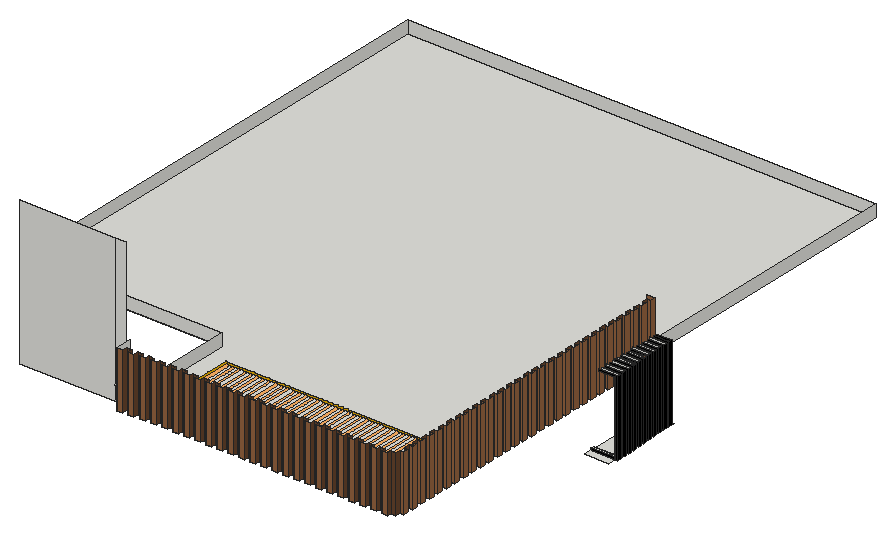
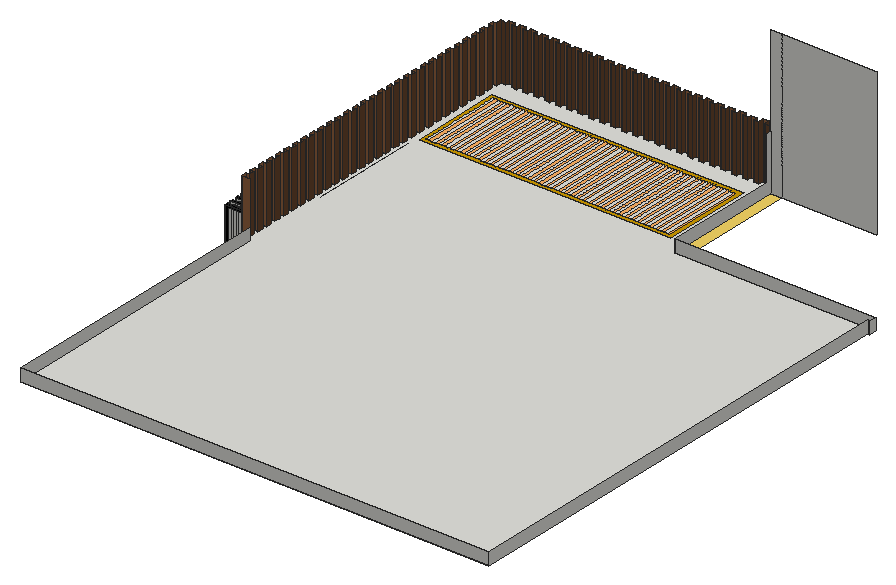
# SketchUp Ruby script. Lengths in inches.
U = 1.inch
M = Sketchup.active_model
def pt(a) = Geom::Point3d.new(a.map { |v| v * U })
def face(e, loops, mat)
  f = e.add_face(loops[0].map { |a| pt(a) })
  loops[1..].each { |l| e.add_face(l.map { |a| pt(a) }).erase! }
  f.material = f.back_material = mat if mat
  f
end
# faces: each face lists its corners as indices into pts; further lists are holes
def faces(e, pts, list, mat = nil) = list.each { |f| face(e, (f[0].is_a?(Array) ? f : [f]).map { |l| l.map { |i| pts[i] } }, mat) }
# xy, xz, yz: faces in a plane at the given z, y or x. An outline is a flat list of corners, or four numbers for a rectangle; further outlines are holes
def ring(l) = l.size == 4 ? [[l[0], l[1]], [l[2], l[1]], [l[2], l[3]], [l[0], l[3]]] : l.each_slice(2).to_a
def flat(e, list, mat, &to3) = list.each { |f| face(e, (f[0].is_a?(Array) ? f : [f]).map { |l| ring(l).map { |u, v| to3.(u, v) } }, mat) }
def xy(e, z, list, mat = nil) = flat(e, list, mat) { |x, y| [x, y, z] }
def xz(e, y, list, mat = nil) = flat(e, list, mat) { |x, z| [x, y, z] }
def yz(e, x, list, mat = nil) = flat(e, list, mat) { |y, z| [x, y, z] }
def lines(e, pts, list) = list.each { |a, b| e.add_line(pt(pts[a]), pt(pts[b])) }
# prism: a flat outline (further loops are holes) pulled along v
def prism(e, loops, v, mat = nil)
  f = face(e, loops, mat); d = Geom::Vector3d.new(v.map { |x| x * U })
  f.pushpull(f.normal.samedirection?(d) ? d.length : -d.length)
end
def box(e, o, s, mat = nil) = prism(e, [[o, [o[0] + s[0], o[1], o[2]], [o[0] + s[0], o[1] + s[1], o[2]], [o[0], o[1] + s[1], o[2]]]], [0, 0, s[2]], mat)
def at(x, y, z, deg = 0) = Geom::Transformation.translation(pt([x, y, z])) * Geom::Transformation.rotation(ORIGIN, Z_AXIS, deg.degrees)
def axes(o, x, y, z) = Geom::Transformation.new([*x, 0, *y, 0, *z, 0, *pt(o).to_a, 1])
def part(name) = M.definitions.add(name)
# library, detail: a bought-in or finely detailed component or shape, given as its bounding box
def library(name, o, s) = part(name).tap { |d| box(d.entities, o, s) }
def detail(e, o, s) = box(e.add_group.entities, o, s)
def put(e, d, t, mat = nil) = e.add_instance(d, t).tap { |i| i.material = mat if mat }
def group(e, t, mat = nil) = e.add_group.tap { |g| g.transformation = t; g.material = mat if mat }.entities
root = M.entities
M.materials.add("C03_Honey_Glow").color = [255, 178, 101]
M.materials.add("D06_Sunflower_Bright").color = [204, 153, 0]
M.materials.add("Glass_Mirror_3").color = [244, 212, 100]
M.materials.add("M09_Shadow_Night").color = [0, 0, 0]
M.materials.add("Wood_Veneer_15_1K").color = [150, 100, 65]
M.materials.add("Wood_Veneer_15_1K1").color = [103, 69, 45]
xy(root,467.31,[[444,372.3125,463.47,378.77],[463.47,378.77,466.08,381.22],[444,381.22,463.47,381.22,463.47,384.31,463.21,384.31,463.21,386.76,463.47,386.76,463.47,389.85,462.95,389.85,462.95,392.29,463.47,392.29,463.47,395.39,462.69,395.39,462.69,397.83,463.47,397.83,463.47,400.92,462.43,400.92,462.43,403.37,463.47,403.37,463.47,406.46,462.17,406.46,462.17,408.91,463.47,408.91,463.47,412,461.91,412,461.91,414.45,463.47,414.45,463.47,417.54,461.65,417.54,461.65,419.99,463.47,419.99,463.47,423.08,461.39,423.08,461.39,425.52,463.47,425.52,463.47,428.62,461.125,428.62,461.125,431.0625,463.47,431.0625,463.47,434.15,460.87,434.15,460.87,436.6,463.47,436.6,463.47,438.64,444,438.64],[463.21,384.31,463.47,386.76],[463.47,384.31,465.82,386.76],
  [462.95,389.85,463.47,392.29],[463.47,389.85,465.56,392.29],[462.69,395.39,463.47,397.83],[463.47,395.39,465.3,397.83],[462.43,400.92,463.47,403.37],
  [463.47,400.92,465.04,403.37],[462.17,406.46,463.47,408.91],[463.47,406.46,464.78,408.91],[461.91,412,463.47,414.45],[463.47,412,464.51,414.45],
  [461.65,417.54,463.47,419.99],[463.47,417.54,464.25,419.99],[461.39,423.08,463.47,425.52],[463.47,423.08,463.99,425.52],[461.125,428.62,463.47,431.0625],
  [463.47,428.62,463.73,431.0625],[460.87,434.15,463.47,436.6]])
xy(root,468.96,[[444,378.77,463.47,381.22]])
xy(root,509.54,[[[222,171,222,278.44,57.3,278.44,57.3,284.23,59.5,284.23,59.5,671.23,443.5,671.23,443.5,436.68,449.91,436.68,449.91,432.33,446.91,432.33,446.91,427.97,449.91,427.97,449.91,423.61,446.91,423.61,446.91,419.25,449.91,419.25,449.91,414.89,446.91,414.89,446.91,410.54,449.91,410.54,449.91,406.18,446.91,406.18,446.91,401.82,449.91,401.82,449.91,397.46,446.91,397.46,446.91,393.11,449.91,393.11,449.91,388.75,446.91,388.75,446.91,384.39,449.91,384.39,449.91,380.03,446.91,380.03,446.91,375.68,449.91,375.68,449.91,371.32,446.91,371.32,446.91,366.96,449.91,366.96,449.91,362.6,446.91,362.6,446.91,358.25,449.91,358.25,449.91,353.89,446.91,353.89,446.91,349.53,449.91,349.53,449.91,345.17,446.91,345.17,446.91,340.82,449.91,340.82,449.91,336.46,446.91,336.46,446.91,332.1,449.91,332.1,449.91,327.74,446.91,327.74,446.91,323.38,449.91,323.38,449.91,319.03,446.91,319.03,446.91,314.67,449.91,314.67,449.91,310.3125,446.91,310.3125,446.91,305.95,449.91,305.95,449.91,301.6,446.91,301.6,446.91,297.24,449.91,297.24,449.91,292.88,446.91,292.88,446.91,288.52,449.91,288.52,449.91,284.17,446.91,284.17,446.91,279.81,449.91,279.81,449.91,275.45,446.91,275.45,446.91,271.09,449.91,271.09,449.91,266.74,446.91,266.74,446.91,262.38,449.91,262.38,449.91,258.02,446.91,258.02,446.91,253.66,449.91,253.66,449.91,249.31,446.91,249.31,446.91,244.95,449.91,244.95,449.91,240.59,446.91,240.59,446.91,236.23,449.91,236.23,449.91,231.875,446.91,231.875,446.91,227.52,449.91,227.52,449.91,223.16,446.91,223.16,446.91,218.8,449.91,218.8,449.91,214.44,446.91,214.44,446.91,210.09,449.91,210.09,449.91,205.73,446.91,205.73,446.91,201.37,449.91,201.37,449.91,197.01,446.91,197.01,446.91,192.66,449.91,192.66,449.91,188.3,446.91,188.3,446.91,183.94,449.91,183.94,449.91,179.58,446.91,179.58,446.91,175.23,442.41,175.23,442.41,172.23,437.91,172.23,437.91,175.23,433.42,175.23,433.42,172.23,428.92,172.23,428.92,175.23,424.42,175.23,424.42,172.23,419.92,172.23,419.92,175.23,415.42,175.23,415.42,172.23,410.92,172.23,410.92,175.23,406.43,175.23,406.43,172.23,401.93,172.23,401.93,175.23,397.43,175.23,397.43,172.23,392.93,172.23,392.93,175.23,388.43,175.23,388.43,172.23,383.9375,172.23,383.9375,175.23,379.4375,175.23,379.4375,172.23,374.9375,172.23,374.9375,175.23,370.44,175.23,370.44,172.23,365.94,172.23,365.94,175.23,361.44,175.23,361.44,172.23,356.95,172.23,356.95,175.23,352.45,175.23,352.45,172.23,347.95,172.23,347.95,175.23,343.45,175.23,343.45,172.23,338.95,172.23,338.95,175.23,334.46,175.23,334.46,172.23,329.96,172.23,329.96,175.23,325.46,175.23,325.46,172.23,320.96,172.23,320.96,175.23,316.46,175.23,316.46,172.23,311.96,172.23,311.96,175.23,307.47,175.23,307.47,172.23,302.97,172.23,302.97,175.23,298.47,175.23,298.47,172.23,293.97,172.23,293.97,175.23,289.47,175.23,289.47,172.23,284.97,172.23,284.97,175.23,280.48,175.23,280.48,172.23,275.98,172.23,275.98,175.23,271.48,175.23,271.48,172.23,266.98,172.23,266.98,175.23,262.48,175.23,262.48,172.23,257.99,172.23,257.99,175.23,253.49,175.23,253.49,172.23,248.99,172.23,248.99,175.23,244.49,175.23,244.49,172.23,239.99,172.23,239.99,175.23,235.49,175.23,235.49,171,231,171,231,175.23,226.5,175.23,226.5,171],[235.75,190.61,441.53,265.07]],[241.25,193.61,243.74,262.07],[246.24,193.61,248.74,262.07],[251.24,193.61,253.73,262.07],[256.23,193.61,258.73,262.07],
  [261.22,193.61,263.72,262.07],[266.22,193.61,268.72,262.07],[271.21,193.61,273.71,262.07],[276.21,193.61,278.71,262.07],[281.2,193.61,283.7,262.07],
  [286.2,193.61,288.69,262.07],[291.19,193.61,293.6875,262.07],[296.1875,193.61,298.68,262.07],[301.18,193.61,303.68,262.07],[306.17,193.61,308.67,262.07],
  [311.17,193.61,313.67,262.07],[316.16,193.61,318.66,262.07],[321.16,193.61,323.65,262.07],[326.15,193.61,328.65,262.07],[331.15,193.61,333.64,262.07],
  [336.14,193.61,338.64,262.07],[341.14,193.61,343.63,262.07],[346.13,193.61,348.625,262.07],[351.125,193.61,353.62,262.07],[356.12,193.61,358.62,262.07],
  [361.11,193.61,363.61,262.07],[366.11,193.61,368.6,262.07],[371.1,193.61,373.6,262.07],[376.1,193.61,378.59,262.07],[381.09,193.61,383.59,262.07],
  [386.09,193.61,388.58,262.07],[391.08,193.61,393.58,262.07],[396.07,193.61,398.57,262.07],[401.07,193.61,403.57,262.07],[406.0625,193.61,408.56,262.07],
  [411.06,193.61,413.55,262.07],[416.05,193.61,418.55,262.07],[421.05,193.61,423.54,262.07],[426.04,193.61,428.54,262.07],[431.03,193.61,433.53,262.07],
  [436.03,193.61,438.53,262.07]])
xy(root,509.54,[[238.75,193.61,241.25,262.07],[243.74,193.61,246.24,262.07],[248.74,193.61,251.24,262.07],[253.73,193.61,256.23,262.07],[258.73,193.61,261.22,262.07],
  [263.72,193.61,266.22,262.07],[268.72,193.61,271.21,262.07],[273.71,193.61,276.21,262.07],[278.71,193.61,281.2,262.07],[283.7,193.61,286.2,262.07],
  [288.69,193.61,291.19,262.07],[293.6875,193.61,296.1875,262.07],[298.68,193.61,301.18,262.07],[303.68,193.61,306.17,262.07],[308.67,193.61,311.17,262.07],
  [313.67,193.61,316.16,262.07],[318.66,193.61,321.16,262.07],[323.65,193.61,326.15,262.07],[328.65,193.61,331.15,262.07],[333.64,193.61,336.14,262.07],
  [338.64,193.61,341.14,262.07],[343.63,193.61,346.13,262.07],[348.625,193.61,351.125,262.07],[353.62,193.61,356.12,262.07],[358.62,193.61,361.11,262.07],
  [363.61,193.61,366.11,262.07],[368.6,193.61,371.1,262.07],[373.6,193.61,376.1,262.07],[378.59,193.61,381.09,262.07],[383.59,193.61,386.09,262.07],
  [388.58,193.61,391.08,262.07],[393.58,193.61,396.07,262.07],[398.57,193.61,401.07,262.07],[403.57,193.61,406.0625,262.07],[408.56,193.61,411.06,262.07],
  [413.55,193.61,416.05,262.07],[418.55,193.61,421.05,262.07],[423.54,193.61,426.04,262.07],[428.54,193.61,431.03,262.07],[433.53,193.61,436.03,262.07]],"C03_Honey_Glow")
xy(root,509.54,[[[235.75,190.61,441.53,265.07],[238.75,193.61,438.53,262.07]]],"D06_Sunflower_Bright")
xy(root,509.54,[[213,180,222,272.89]],"Glass_Mirror_3")
xz(root,171,[[222,509.54,226.5,555.54],[231,509.54,235.49,555.54]],"Wood_Veneer_15_1K")
xz(root,172.23,[[239.99,509.54,244.49,555.54],[248.99,509.54,253.49,555.54],[257.99,509.54,262.48,555.54],[266.98,509.54,271.48,555.54],[275.98,509.54,280.48,555.54],
  [284.97,509.54,289.47,555.54],[293.97,509.54,298.47,555.54],[302.97,509.54,307.47,555.54],[311.96,509.54,316.46,555.54],[320.96,509.54,325.46,555.54],
  [329.96,509.54,334.46,555.54],[338.95,509.54,343.45,555.54],[347.95,509.54,352.45,555.54],[356.95,509.54,361.44,555.54],[365.94,509.54,370.44,555.54],
  [374.9375,509.54,379.4375,555.54],[383.9375,509.54,388.43,555.54],[392.93,509.54,397.43,555.54],[401.93,509.54,406.43,555.54],[410.92,509.54,415.42,555.54],
  [419.92,509.54,424.42,555.54],[428.92,509.54,433.42,555.54],[437.91,509.54,442.41,555.54]],"Wood_Veneer_15_1K")
xz(root,175.23,[[226.5,509.54,231,555.54],[235.49,509.54,239.99,555.54],[244.49,509.54,248.99,555.54],[253.49,509.54,257.99,555.54],[262.48,509.54,266.98,555.54],
  [271.48,509.54,275.98,555.54],[280.48,509.54,284.97,555.54],[289.47,509.54,293.97,555.54],[298.47,509.54,302.97,555.54],[307.47,509.54,311.96,555.54],
  [316.46,509.54,320.96,555.54],[325.46,509.54,329.96,555.54],[334.46,509.54,338.95,555.54],[343.45,509.54,347.95,555.54],[352.45,509.54,356.95,555.54],
  [361.44,509.54,365.94,555.54],[370.44,509.54,374.9375,555.54],[379.4375,509.54,383.9375,555.54],[388.43,509.54,392.93,555.54],[397.43,509.54,401.93,555.54],
  [406.43,509.54,410.92,555.54],[415.42,509.54,419.92,555.54],[424.42,509.54,428.92,555.54],[433.42,509.54,437.91,555.54],[442.41,509.54,446.91,555.54]],"Wood_Veneer_15_1K1")
xz(root,179.58,[[446.91,509.54,449.91,555.54]],"Wood_Veneer_15_1K")
xz(root,180,[[135.55,509.54,213,629.54],[213,509.54,222,629.54]])
xz(root,183.94,[[446.91,509.54,449.91,555.54]],"Wood_Veneer_15_1K")
xz(root,188.3,[[446.91,509.54,449.91,555.54]],"Wood_Veneer_15_1K")
xz(root,192.66,[[446.91,509.54,449.91,555.54]],"Wood_Veneer_15_1K")
xz(root,197.01,[[446.91,509.54,449.91,555.54]],"Wood_Veneer_15_1K")
xz(root,201.37,[[446.91,509.54,449.91,555.54]],"Wood_Veneer_15_1K")
xz(root,205.73,[[446.91,509.54,449.91,555.54]],"Wood_Veneer_15_1K")
xz(root,210.09,[[446.91,509.54,449.91,555.54]],"Wood_Veneer_15_1K")
xz(root,214.44,[[446.91,509.54,449.91,555.54]],"Wood_Veneer_15_1K")
xz(root,218.8,[[446.91,509.54,449.91,555.54]],"Wood_Veneer_15_1K")
xz(root,223.16,[[446.91,509.54,449.91,555.54]],"Wood_Veneer_15_1K")
xz(root,227.52,[[446.91,509.54,449.91,555.54]],"Wood_Veneer_15_1K")
xz(root,231.875,[[446.91,509.54,449.91,555.54]],"Wood_Veneer_15_1K")
xz(root,236.23,[[446.91,509.54,449.91,555.54]],"Wood_Veneer_15_1K")
xz(root,240.59,[[446.91,509.54,449.91,555.54]],"Wood_Veneer_15_1K")
xz(root,244.95,[[446.91,509.54,449.91,555.54]],"Wood_Veneer_15_1K")
xz(root,249.31,[[446.91,509.54,449.91,555.54]],"Wood_Veneer_15_1K")
xz(root,253.66,[[446.91,509.54,449.91,555.54]],"Wood_Veneer_15_1K")
xz(root,258.02,[[446.91,509.54,449.91,555.54]],"Wood_Veneer_15_1K")
xz(root,262.38,[[446.91,509.54,449.91,555.54]],"Wood_Veneer_15_1K")
xz(root,266.74,[[446.91,509.54,449.91,555.54]],"Wood_Veneer_15_1K")
xz(root,271.09,[[446.91,509.54,449.91,555.54]],"Wood_Veneer_15_1K")
xz(root,275.45,[[446.91,509.54,449.91,555.54]],"Wood_Veneer_15_1K")
xz(root,278.44,[[57.3,509.54,222,519.54]])
xz(root,279.81,[[446.91,509.54,449.91,555.54]],"Wood_Veneer_15_1K")
xz(root,284.17,[[446.91,509.54,449.91,555.54]],"Wood_Veneer_15_1K")
xz(root,284.23,[[57.3,509.54,59.5,519.54]])
xz(root,288.52,[[446.91,509.54,449.91,555.54]],"Wood_Veneer_15_1K")
xz(root,292.88,[[446.91,509.54,449.91,555.54]],"Wood_Veneer_15_1K")
xz(root,297.24,[[446.91,509.54,449.91,555.54]],"Wood_Veneer_15_1K")
xz(root,301.6,[[446.91,509.54,449.91,555.54]],"Wood_Veneer_15_1K")
xz(root,305.95,[[446.91,509.54,449.91,555.54]],"Wood_Veneer_15_1K")
xz(root,310.3125,[[446.91,509.54,449.91,555.54]],"Wood_Veneer_15_1K")
xz(root,314.67,[[446.91,509.54,449.91,555.54]],"Wood_Veneer_15_1K")
xz(root,319.03,[[446.91,509.54,449.91,555.54]],"Wood_Veneer_15_1K")
xz(root,323.38,[[446.91,509.54,449.91,555.54]],"Wood_Veneer_15_1K")
xz(root,327.74,[[446.91,509.54,449.91,555.54]],"Wood_Veneer_15_1K")
xz(root,332.1,[[446.91,509.54,449.91,555.54]],"Wood_Veneer_15_1K")
xz(root,336.46,[[446.91,509.54,449.91,555.54]],"Wood_Veneer_15_1K")
xz(root,340.82,[[446.91,509.54,449.91,555.54]],"Wood_Veneer_15_1K")
xz(root,345.17,[[446.91,509.54,449.91,555.54]],"Wood_Veneer_15_1K")
xz(root,349.53,[[446.91,509.54,449.91,555.54]],"Wood_Veneer_15_1K")
xz(root,353.89,[[446.91,509.54,449.91,555.54]],"Wood_Veneer_15_1K")
xz(root,358.25,[[446.91,509.54,449.91,555.54]],"Wood_Veneer_15_1K")
xz(root,362.6,[[446.91,509.54,449.91,555.54]],"Wood_Veneer_15_1K")
xz(root,366.96,[[446.91,509.54,449.91,555.54]],"Wood_Veneer_15_1K")
xz(root,371.32,[[446.91,509.54,449.91,555.54]],"Wood_Veneer_15_1K")
xz(root,375.68,[[446.91,509.54,449.91,555.54]],"Wood_Veneer_15_1K")
xz(root,378.77,[[444,467.31,463.47,468.96],[463.47,467.31,466.08,467.31,466.08,529.36,449.91,529.36,449.91,527.89,463.47,527.89]],"M09_Shadow_Night")
xz(root,380.03,[[446.91,509.54,449.91,555.54]],"Wood_Veneer_15_1K")
xz(root,381.22,[[444,467.31,463.47,468.96],[463.47,467.31,463.47,527.89,449.91,527.89,449.91,529.36,466.08,529.36,466.08,467.31]])
xz(root,384.31,[[463.21,467.31,465.82,467.31,465.82,529.36,449.91,529.36,449.91,527.89,463.21,527.89]],"M09_Shadow_Night")
xz(root,384.39,[[446.91,509.54,449.91,555.54]],"Wood_Veneer_15_1K")
xz(root,386.76,[[463.21,467.31,463.21,527.89,449.91,527.89,449.91,529.36,465.82,529.36,465.82,467.31]])
xz(root,388.75,[[446.91,509.54,449.91,555.54]],"Wood_Veneer_15_1K")
xz(root,389.85,[[462.95,467.31,465.56,467.31,465.56,529.36,449.91,529.36,449.91,527.89,462.95,527.89]],"M09_Shadow_Night")
xz(root,392.29,[[462.95,467.31,462.95,527.89,449.91,527.89,449.91,529.36,465.56,529.36,465.56,467.31]])
xz(root,393.11,[[446.91,509.54,449.91,555.54]],"Wood_Veneer_15_1K")
xz(root,395.39,[[462.69,467.31,465.3,467.31,465.3,529.36,449.91,529.36,449.91,527.89,462.69,527.89]],"M09_Shadow_Night")
xz(root,397.46,[[446.91,509.54,449.91,555.54]],"Wood_Veneer_15_1K")
xz(root,397.83,[[462.69,467.31,462.69,527.89,449.91,527.89,449.91,529.36,465.3,529.36,465.3,467.31]])
xz(root,400.92,[[462.43,467.31,465.04,467.31,465.04,529.36,449.91,529.36,449.91,527.89,462.43,527.89]],"M09_Shadow_Night")
xz(root,401.82,[[446.91,509.54,449.91,555.54]],"Wood_Veneer_15_1K")
xz(root,403.37,[[462.43,467.31,462.43,527.89,449.91,527.89,449.91,529.36,465.04,529.36,465.04,467.31]])
xz(root,406.18,[[446.91,509.54,449.91,555.54]],"Wood_Veneer_15_1K")
xz(root,406.46,[[462.17,467.31,464.78,467.31,464.78,529.36,449.91,529.36,449.91,527.89,462.17,527.89]],"M09_Shadow_Night")
xz(root,408.91,[[462.17,467.31,462.17,527.89,449.91,527.89,449.91,529.36,464.78,529.36,464.78,467.31]])
xz(root,410.54,[[446.91,509.54,449.91,555.54]],"Wood_Veneer_15_1K")
xz(root,412,[[461.91,467.31,464.51,467.31,464.51,529.36,449.91,529.36,449.91,527.89,461.91,527.89]],"M09_Shadow_Night")
xz(root,414.45,[[461.91,467.31,461.91,527.89,449.91,527.89,449.91,529.36,464.51,529.36,464.51,467.31]])
xz(root,414.89,[[446.91,509.54,449.91,555.54]],"Wood_Veneer_15_1K")
xz(root,417.54,[[461.65,467.31,464.25,467.31,464.25,529.36,449.91,529.36,449.91,527.89,461.65,527.89]],"M09_Shadow_Night")
xz(root,419.25,[[446.91,509.54,449.91,555.54]],"Wood_Veneer_15_1K")
xz(root,419.99,[[461.65,467.31,461.65,527.89,449.91,527.89,449.91,529.36,464.25,529.36,464.25,467.31]])
xz(root,423.08,[[461.39,467.31,463.99,467.31,463.99,529.36,449.91,529.36,449.91,527.89,461.39,527.89]],"M09_Shadow_Night")
xz(root,423.61,[[446.91,509.54,449.91,555.54]],"Wood_Veneer_15_1K")
xz(root,425.52,[[461.39,467.31,461.39,527.89,449.91,527.89,449.91,529.36,463.99,529.36,463.99,467.31]])
xz(root,427.97,[[446.91,509.54,449.91,555.54]],"Wood_Veneer_15_1K")
xz(root,428.62,[[461.125,467.31,463.73,467.31,463.73,529.36,449.91,529.36,449.91,527.89,461.125,527.89]],"M09_Shadow_Night")
xz(root,431.0625,[[461.125,467.31,461.125,527.89,449.91,527.89,449.91,529.36,463.73,529.36,463.73,467.31]])
xz(root,432.33,[[446.91,509.54,449.91,555.54]],"Wood_Veneer_15_1K")
xz(root,434.15,[[460.87,467.31,463.47,467.31,463.47,529.36,449.91,529.36,449.91,527.89,460.87,527.89]],"M09_Shadow_Night")
xz(root,436.6,[[460.87,467.31,460.87,527.89,449.91,527.89,449.91,529.36,463.47,529.36,463.47,467.31]],"M09_Shadow_Night")
xz(root,436.68,[[443.5,509.54,449.91,555.54]],"Wood_Veneer_15_1K")
xz(root,671.23,[[59.5,509.54,443.5,519.54]])
yz(root,57.3,[[278.44,509.54,284.23,519.54]])
yz(root,59.5,[[284.23,509.54,671.23,519.54]])
yz(root,222,[[171,509.54,171,555.54,184.49,555.54,184.49,519.54,278.44,519.54,278.44,509.54]])
yz(root,226.5,[[171,509.54,175.23,555.54]],"Wood_Veneer_15_1K1")
yz(root,231,[[171,509.54,175.23,555.54]],"Wood_Veneer_15_1K1")
yz(root,235.49,[[171,509.54,175.23,555.54]],"Wood_Veneer_15_1K1")
yz(root,239.99,[[172.23,509.54,175.23,555.54]],"Wood_Veneer_15_1K1")
yz(root,244.49,[[172.23,509.54,175.23,555.54]],"Wood_Veneer_15_1K1")
yz(root,248.99,[[172.23,509.54,175.23,555.54]],"Wood_Veneer_15_1K1")
yz(root,253.49,[[172.23,509.54,175.23,555.54]],"Wood_Veneer_15_1K1")
yz(root,257.99,[[172.23,509.54,175.23,555.54]],"Wood_Veneer_15_1K1")
yz(root,262.48,[[172.23,509.54,175.23,555.54]],"Wood_Veneer_15_1K1")
yz(root,266.98,[[172.23,509.54,175.23,555.54]],"Wood_Veneer_15_1K1")
yz(root,271.48,[[172.23,509.54,175.23,555.54]],"Wood_Veneer_15_1K1")
yz(root,275.98,[[172.23,509.54,175.23,555.54]],"Wood_Veneer_15_1K1")
yz(root,280.48,[[172.23,509.54,175.23,555.54]],"Wood_Veneer_15_1K1")
yz(root,284.97,[[172.23,509.54,175.23,555.54]],"Wood_Veneer_15_1K1")
yz(root,289.47,[[172.23,509.54,175.23,555.54]],"Wood_Veneer_15_1K1")
yz(root,293.97,[[172.23,509.54,175.23,555.54]],"Wood_Veneer_15_1K1")
yz(root,298.47,[[172.23,509.54,175.23,555.54]],"Wood_Veneer_15_1K1")
yz(root,302.97,[[172.23,509.54,175.23,555.54]],"Wood_Veneer_15_1K1")
yz(root,307.47,[[172.23,509.54,175.23,555.54]],"Wood_Veneer_15_1K1")
yz(root,311.96,[[172.23,509.54,175.23,555.54]],"Wood_Veneer_15_1K1")
yz(root,316.46,[[172.23,509.54,175.23,555.54]],"Wood_Veneer_15_1K1")
yz(root,320.96,[[172.23,509.54,175.23,555.54]],"Wood_Veneer_15_1K1")
yz(root,325.46,[[172.23,509.54,175.23,555.54]],"Wood_Veneer_15_1K1")
yz(root,329.96,[[172.23,509.54,175.23,555.54]],"Wood_Veneer_15_1K1")
yz(root,334.46,[[172.23,509.54,175.23,555.54]],"Wood_Veneer_15_1K1")
yz(root,338.95,[[172.23,509.54,175.23,555.54]],"Wood_Veneer_15_1K1")
yz(root,343.45,[[172.23,509.54,175.23,555.54]],"Wood_Veneer_15_1K1")
yz(root,347.95,[[172.23,509.54,175.23,555.54]],"Wood_Veneer_15_1K1")
yz(root,352.45,[[172.23,509.54,175.23,555.54]],"Wood_Veneer_15_1K1")
yz(root,356.95,[[172.23,509.54,175.23,555.54]],"Wood_Veneer_15_1K1")
yz(root,361.44,[[172.23,509.54,175.23,555.54]],"Wood_Veneer_15_1K1")
yz(root,365.94,[[172.23,509.54,175.23,555.54]],"Wood_Veneer_15_1K1")
yz(root,370.44,[[172.23,509.54,175.23,555.54]],"Wood_Veneer_15_1K1")
yz(root,374.9375,[[172.23,509.54,175.23,555.54]],"Wood_Veneer_15_1K1")
yz(root,379.4375,[[172.23,509.54,175.23,555.54]],"Wood_Veneer_15_1K1")
yz(root,383.9375,[[172.23,509.54,175.23,555.54]],"Wood_Veneer_15_1K1")
yz(root,388.43,[[172.23,509.54,175.23,555.54]],"Wood_Veneer_15_1K1")
yz(root,392.93,[[172.23,509.54,175.23,555.54]],"Wood_Veneer_15_1K1")
yz(root,397.43,[[172.23,509.54,175.23,555.54]],"Wood_Veneer_15_1K1")
yz(root,401.93,[[172.23,509.54,175.23,555.54]],"Wood_Veneer_15_1K1")
yz(root,406.43,[[172.23,509.54,175.23,555.54]],"Wood_Veneer_15_1K1")
yz(root,410.92,[[172.23,509.54,175.23,555.54]],"Wood_Veneer_15_1K1")
yz(root,415.42,[[172.23,509.54,175.23,555.54]],"Wood_Veneer_15_1K1")
yz(root,419.92,[[172.23,509.54,175.23,555.54]],"Wood_Veneer_15_1K1")
yz(root,424.42,[[172.23,509.54,175.23,555.54]],"Wood_Veneer_15_1K1")
yz(root,428.92,[[172.23,509.54,175.23,555.54]],"Wood_Veneer_15_1K1")
yz(root,433.42,[[172.23,509.54,175.23,555.54]],"Wood_Veneer_15_1K1")
yz(root,437.91,[[172.23,509.54,175.23,555.54]],"Wood_Veneer_15_1K1")
yz(root,442.41,[[172.23,509.54,175.23,555.54]],"Wood_Veneer_15_1K1")
yz(root,443.5,[[436.68,509.54,671.23,519.54]])
yz(root,446.91,[[175.23,509.54,179.58,555.54],[183.94,509.54,188.3,555.54],[192.66,509.54,197.01,555.54],[201.37,509.54,205.73,555.54],[210.09,509.54,214.44,555.54],
  [218.8,509.54,223.16,555.54],[227.52,509.54,231.875,555.54],[236.23,509.54,240.59,555.54],[244.95,509.54,249.31,555.54],[253.66,509.54,258.02,555.54],
  [262.38,509.54,266.74,555.54],[271.09,509.54,275.45,555.54],[279.81,509.54,284.17,555.54],[288.52,509.54,292.88,555.54],[297.24,509.54,301.6,555.54],
  [305.95,509.54,310.3125,555.54],[314.67,509.54,319.03,555.54],[323.38,509.54,327.74,555.54],[332.1,509.54,336.46,555.54],[340.82,509.54,345.17,555.54],
  [349.53,509.54,353.89,555.54],[358.25,509.54,362.6,555.54],[366.96,509.54,371.32,555.54],[375.68,509.54,380.03,555.54],[384.39,509.54,388.75,555.54],
  [393.11,509.54,397.46,555.54],[401.82,509.54,406.18,555.54],[410.54,509.54,414.89,555.54],[419.25,509.54,423.61,555.54],[427.97,509.54,432.33,555.54]],"Wood_Veneer_15_1K1")
yz(root,449.91,[[179.58,509.54,183.94,555.54],[188.3,509.54,192.66,555.54],[197.01,509.54,201.37,555.54],[205.73,509.54,210.09,555.54],[214.44,509.54,218.8,555.54],
  [223.16,509.54,227.52,555.54],[231.875,509.54,236.23,555.54],[240.59,509.54,244.95,555.54],[249.31,509.54,253.66,555.54],[258.02,509.54,262.38,555.54],
  [266.74,509.54,271.09,555.54],[275.45,509.54,279.81,555.54],[284.17,509.54,288.52,555.54],[292.88,509.54,297.24,555.54],[301.6,509.54,305.95,555.54],
  [310.3125,509.54,314.67,555.54],[319.03,509.54,323.38,555.54],[327.74,509.54,332.1,555.54],[336.46,509.54,340.82,555.54],[345.17,509.54,349.53,555.54],
  [353.89,509.54,358.25,555.54],[362.6,509.54,366.96,555.54],[371.32,509.54,375.68,555.54],[380.03,509.54,384.39,555.54],[388.75,509.54,393.11,555.54],
  [397.46,509.54,401.82,555.54],[406.18,509.54,410.54,555.54],[414.89,509.54,419.25,555.54],[423.61,509.54,427.97,555.54],[432.33,509.54,436.68,555.54]],"Wood_Veneer_15_1K")
yz(root,460.87,[[434.15,467.31,436.6,527.89]])
yz(root,461.125,[[428.62,467.31,431.0625,527.89]])
yz(root,461.39,[[423.08,467.31,425.52,527.89]])
yz(root,461.65,[[417.54,467.31,419.99,527.89]])
yz(root,461.91,[[412,467.31,414.45,527.89]])
yz(root,462.17,[[406.46,467.31,408.91,527.89]])
yz(root,462.43,[[400.92,467.31,403.37,527.89]])
yz(root,462.69,[[395.39,467.31,397.83,527.89]])
yz(root,462.95,[[389.85,467.31,392.29,527.89]])
yz(root,463.21,[[384.31,467.31,386.76,527.89]])
yz(root,463.47,[[378.77,467.31,381.22,468.96],[378.77,468.96,381.22,527.89]])
yz(root,463.47,[[434.15,467.31,436.6,529.36]],"M09_Shadow_Night")
yz(root,463.73,[[428.62,467.31,431.0625,529.36]],"M09_Shadow_Night")
yz(root,463.99,[[423.08,467.31,425.52,529.36]],"M09_Shadow_Night")
yz(root,464.25,[[417.54,467.31,419.99,529.36]],"M09_Shadow_Night")
yz(root,464.51,[[412,467.31,414.45,529.36]],"M09_Shadow_Night")
yz(root,464.78,[[406.46,467.31,408.91,529.36]],"M09_Shadow_Night")
yz(root,465.04,[[400.92,467.31,403.37,529.36]],"M09_Shadow_Night")
yz(root,465.3,[[395.39,467.31,397.83,529.36]],"M09_Shadow_Night")
yz(root,465.56,[[389.85,467.31,392.29,529.36]],"M09_Shadow_Night")
yz(root,465.82,[[384.31,467.31,386.76,529.36]],"M09_Shadow_Night")
yz(root,466.08,[[378.77,467.31,381.22,529.36]],"M09_Shadow_Night")
p = [[444,273.3,509.69],[444,351.82,509.69],[444,363.42,509.69]]
lines(root,p,[[0,1],[1,2]])
